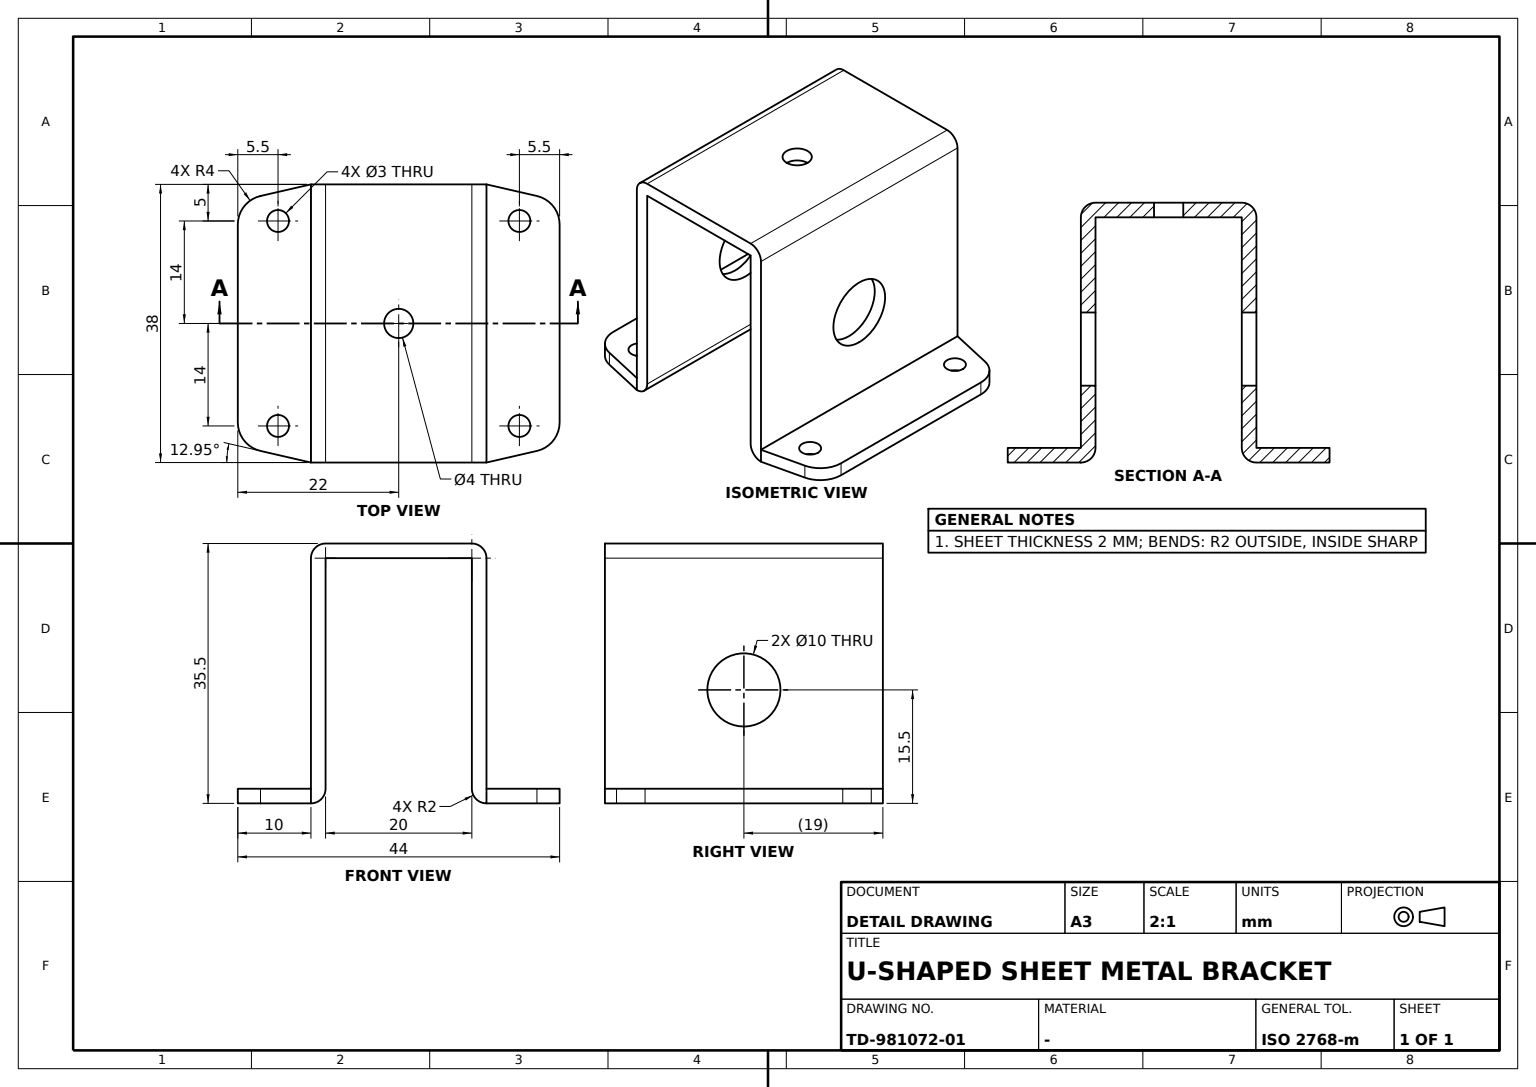
ISO-10303-21;
HEADER;
FILE_DESCRIPTION((''),'2;1');
FILE_NAME('','',(''),(''),'','','');
FILE_SCHEMA(('AUTOMOTIVE_DESIGN'));
ENDSEC;
DATA;
#1=APPLICATION_CONTEXT('');
#2=PRODUCT_CONTEXT('',#1,'mechanical');
#3=PRODUCT('','','',(#2));
#4=PRODUCT_DEFINITION_FORMATION('','',#3);
#5=PRODUCT_DEFINITION_CONTEXT('',#1,'design');
#6=PRODUCT_DEFINITION('','',#4,#5);
#7=PRODUCT_DEFINITION_SHAPE('','',#6);
#8=(LENGTH_UNIT()NAMED_UNIT(*)SI_UNIT(.MILLI.,.METRE.));
#9=(NAMED_UNIT(*)PLANE_ANGLE_UNIT()SI_UNIT($,.RADIAN.));
#10=(NAMED_UNIT(*)SI_UNIT($,.STERADIAN.)SOLID_ANGLE_UNIT());
#11=UNCERTAINTY_MEASURE_WITH_UNIT(LENGTH_MEASURE(0.005),#8,'distance_accuracy_value','');
#12=(GEOMETRIC_REPRESENTATION_CONTEXT(3)GLOBAL_UNCERTAINTY_ASSIGNED_CONTEXT((#11))GLOBAL_UNIT_ASSIGNED_CONTEXT((#8,#9,#10))REPRESENTATION_CONTEXT('',''));
#13=CARTESIAN_POINT('',(-19.,-10.,-31.5));
#14=VERTEX_POINT('',#13);
#15=CARTESIAN_POINT('',(19.,-10.,-31.5));
#16=VERTEX_POINT('',#15);
#17=CARTESIAN_POINT('',(0.,-10.,-31.5));
#18=DIRECTION('',(-1.,0.,0.));
#19=VECTOR('',#18,1000.);
#20=LINE('',#17,#19);
#21=EDGE_CURVE('',#14,#16,#20,.F.);
#22=ORIENTED_EDGE('',*,*,#21,.F.);
#23=CARTESIAN_POINT('',(-19.,-10.,0.));
#24=VERTEX_POINT('',#23);
#25=CARTESIAN_POINT('',(-19.,-10.,2.));
#26=DIRECTION('',(0.,0.,1.));
#27=VECTOR('',#26,1000.);
#28=LINE('',#25,#27);
#29=EDGE_CURVE('',#24,#14,#28,.F.);
#30=ORIENTED_EDGE('',*,*,#29,.F.);
#31=CARTESIAN_POINT('',(19.,-10.,0.));
#32=VERTEX_POINT('',#31);
#33=CARTESIAN_POINT('',(0.,-10.,0.));
#34=DIRECTION('',(1.,0.,0.));
#35=VECTOR('',#34,1000.);
#36=LINE('',#33,#35);
#37=EDGE_CURVE('',#24,#32,#36,.T.);
#38=ORIENTED_EDGE('',*,*,#37,.T.);
#39=CARTESIAN_POINT('',(19.,-10.,2.));
#40=DIRECTION('',(0.,0.,-1.));
#41=VECTOR('',#40,1000.);
#42=LINE('',#39,#41);
#43=EDGE_CURVE('',#32,#16,#42,.T.);
#44=ORIENTED_EDGE('',*,*,#43,.T.);
#45=EDGE_LOOP('',(#22,#30,#38,#44));
#46=FACE_BOUND('',#45,.T.);
#47=CARTESIAN_POINT('',(0.,-10.,-23.));
#48=VERTEX_POINT('',#47);
#49=CARTESIAN_POINT('',(0.,-10.,-18.));
#50=DIRECTION('',(0.,-1.,0.));
#51=AXIS2_PLACEMENT_3D('',#49,#50,#40);
#52=CIRCLE('',#51,5.);
#53=EDGE_CURVE('',#48,#48,#52,.T.);
#54=ORIENTED_EDGE('',*,*,#53,.T.);
#55=EDGE_LOOP('',(#54));
#56=FACE_BOUND('',#55,.T.);
#57=CARTESIAN_POINT('',(0.,-10.,2.));
#58=AXIS2_PLACEMENT_3D('',#57,#50,#18);
#59=PLANE('',#58);
#60=ADVANCED_FACE('',(#46,#56),#59,.F.);
#61=CARTESIAN_POINT('',(-19.,-12.,0.));
#62=VERTEX_POINT('',#61);
#63=VERTEX_POINT('',#25);
#64=AXIS2_PLACEMENT_3D('',#23,#34,#40);
#65=CIRCLE('',#64,2.);
#66=EDGE_CURVE('',#62,#63,#65,.F.);
#67=ORIENTED_EDGE('',*,*,#66,.F.);
#68=CARTESIAN_POINT('',(19.,-12.,0.));
#69=VERTEX_POINT('',#68);
#70=CARTESIAN_POINT('',(0.,-12.,0.));
#71=LINE('',#70,#35);
#72=EDGE_CURVE('',#69,#62,#71,.F.);
#73=ORIENTED_EDGE('',*,*,#72,.F.);
#74=VERTEX_POINT('',#39);
#75=AXIS2_PLACEMENT_3D('',#31,#18,#26);
#76=CIRCLE('',#75,2.);
#77=EDGE_CURVE('',#69,#74,#76,.T.);
#78=ORIENTED_EDGE('',*,*,#77,.T.);
#79=LINE('',#57,#35);
#80=EDGE_CURVE('',#74,#63,#79,.F.);
#81=ORIENTED_EDGE('',*,*,#80,.T.);
#82=EDGE_LOOP('',(#67,#73,#78,#81));
#83=FACE_BOUND('',#82,.T.);
#84=AXIS2_PLACEMENT_3D('',#33,#34,#50);
#85=CYLINDRICAL_SURFACE('',#84,2.);
#86=ADVANCED_FACE('',(#83),#85,.T.);
#87=CARTESIAN_POINT('',(0.,-12.,-23.));
#88=VERTEX_POINT('',#87);
#89=CARTESIAN_POINT('',(0.,-12.,-18.));
#90=AXIS2_PLACEMENT_3D('',#89,#50,#40);
#91=CIRCLE('',#90,5.);
#92=EDGE_CURVE('',#88,#88,#91,.T.);
#93=ORIENTED_EDGE('',*,*,#92,.T.);
#94=EDGE_LOOP('',(#93));
#95=FACE_BOUND('',#94,.T.);
#96=ORIENTED_EDGE('',*,*,#53,.F.);
#97=EDGE_LOOP('',(#96));
#98=FACE_BOUND('',#97,.T.);
#99=CARTESIAN_POINT('',(0.,11.,-18.));
#100=AXIS2_PLACEMENT_3D('',#99,#50,#34);
#101=CYLINDRICAL_SURFACE('',#100,5.);
#102=ADVANCED_FACE('',(#95,#98),#101,.F.);
#103=CARTESIAN_POINT('',(-14.,-15.,-31.5));
#104=VERTEX_POINT('',#103);
#105=CARTESIAN_POINT('',(-14.,-16.5,-31.5));
#106=DIRECTION('',(0.,1.,0.));
#107=AXIS2_PLACEMENT_3D('',#105,#40,#106);
#108=CIRCLE('',#107,1.5);
#109=EDGE_CURVE('',#104,#104,#108,.T.);
#110=ORIENTED_EDGE('',*,*,#109,.F.);
#111=EDGE_LOOP('',(#110));
#112=FACE_BOUND('',#111,.T.);
#113=CARTESIAN_POINT('',(-14.,-15.,-33.5));
#114=VERTEX_POINT('',#113);
#115=CARTESIAN_POINT('',(-14.,-16.5,-33.5));
#116=AXIS2_PLACEMENT_3D('',#115,#40,#106);
#117=CIRCLE('',#116,1.5);
#118=EDGE_CURVE('',#114,#114,#117,.T.);
#119=ORIENTED_EDGE('',*,*,#118,.T.);
#120=EDGE_LOOP('',(#119));
#121=FACE_BOUND('',#120,.T.);
#122=CYLINDRICAL_SURFACE('',#107,1.5);
#123=ADVANCED_FACE('',(#112,#121),#122,.F.);
#124=CARTESIAN_POINT('',(-19.,-12.,-33.5));
#125=VERTEX_POINT('',#124);
#126=CARTESIAN_POINT('',(-19.,-12.,-31.5));
#127=VERTEX_POINT('',#126);
#128=LINE('',#126,#27);
#129=EDGE_CURVE('',#125,#127,#128,.T.);
#130=ORIENTED_EDGE('',*,*,#129,.F.);
#131=CARTESIAN_POINT('',(-17.413784,-18.896591,-33.5));
#132=VERTEX_POINT('',#131);
#133=CARTESIAN_POINT('',(-24.242663,10.794187,-33.5));
#134=DIRECTION('',(-0.224147693,0.974555187,0.));
#135=VECTOR('',#134,1000.);
#136=LINE('',#133,#135);
#137=EDGE_CURVE('',#132,#125,#136,.T.);
#138=ORIENTED_EDGE('',*,*,#137,.F.);
#139=CARTESIAN_POINT('',(-17.413784,-18.896591,-31.5));
#140=VERTEX_POINT('',#139);
#141=LINE('',#131,#41);
#142=EDGE_CURVE('',#132,#140,#141,.F.);
#143=ORIENTED_EDGE('',*,*,#142,.T.);
#144=CARTESIAN_POINT('',(-24.242663,10.794187,-31.5));
#145=LINE('',#144,#135);
#146=EDGE_CURVE('',#140,#127,#145,.T.);
#147=ORIENTED_EDGE('',*,*,#146,.T.);
#148=EDGE_LOOP('',(#130,#138,#143,#147));
#149=FACE_BOUND('',#148,.T.);
#150=CARTESIAN_POINT('',(-17.85,-17.,-31.5));
#151=DIRECTION('',(-0.974555187,-0.224147693,0.));
#152=DIRECTION('',(0.224147693,-0.974555187,0.));
#153=AXIS2_PLACEMENT_3D('',#150,#151,#152);
#154=PLANE('',#153);
#155=ADVANCED_FACE('',(#149),#154,.T.);
#156=CARTESIAN_POINT('',(14.,-15.,-31.5));
#157=VERTEX_POINT('',#156);
#158=CARTESIAN_POINT('',(14.,-16.5,-31.5));
#159=AXIS2_PLACEMENT_3D('',#158,#40,#106);
#160=CIRCLE('',#159,1.5);
#161=EDGE_CURVE('',#157,#157,#160,.F.);
#162=ORIENTED_EDGE('',*,*,#161,.T.);
#163=EDGE_LOOP('',(#162));
#164=FACE_BOUND('',#163,.T.);
#165=CARTESIAN_POINT('',(14.,-15.,-33.5));
#166=VERTEX_POINT('',#165);
#167=CARTESIAN_POINT('',(14.,-16.5,-33.5));
#168=AXIS2_PLACEMENT_3D('',#167,#40,#106);
#169=CIRCLE('',#168,1.5);
#170=EDGE_CURVE('',#166,#166,#169,.F.);
#171=ORIENTED_EDGE('',*,*,#170,.F.);
#172=EDGE_LOOP('',(#171));
#173=FACE_BOUND('',#172,.T.);
#174=CYLINDRICAL_SURFACE('',#159,1.5);
#175=ADVANCED_FACE('',(#164,#173),#174,.F.);
#176=CARTESIAN_POINT('',(13.515563,22.,-33.5));
#177=VERTEX_POINT('',#176);
#178=CARTESIAN_POINT('',(-13.515563,22.,-33.5));
#179=VERTEX_POINT('',#178);
#180=CARTESIAN_POINT('',(-19.,22.,-33.5));
#181=LINE('',#180,#19);
#182=EDGE_CURVE('',#177,#179,#181,.T.);
#183=ORIENTED_EDGE('',*,*,#182,.F.);
#184=CARTESIAN_POINT('',(17.413784,18.896591,-33.5));
#185=VERTEX_POINT('',#184);
#186=CARTESIAN_POINT('',(13.515563,18.,-33.5));
#187=AXIS2_PLACEMENT_3D('',#186,#40,#106);
#188=CIRCLE('',#187,4.);
#189=EDGE_CURVE('',#185,#177,#188,.F.);
#190=ORIENTED_EDGE('',*,*,#189,.F.);
#191=CARTESIAN_POINT('',(19.,12.,-33.5));
#192=VERTEX_POINT('',#191);
#193=CARTESIAN_POINT('',(17.090797,20.300883,-33.5));
#194=VECTOR('',#152,1000.);
#195=LINE('',#193,#194);
#196=EDGE_CURVE('',#185,#192,#195,.T.);
#197=ORIENTED_EDGE('',*,*,#196,.T.);
#198=CARTESIAN_POINT('',(-19.,12.,-33.5));
#199=VERTEX_POINT('',#198);
#200=CARTESIAN_POINT('',(0.,12.,-33.5));
#201=LINE('',#200,#35);
#202=EDGE_CURVE('',#199,#192,#201,.T.);
#203=ORIENTED_EDGE('',*,*,#202,.F.);
#204=CARTESIAN_POINT('',(-17.413784,18.896591,-33.5));
#205=VERTEX_POINT('',#204);
#206=DIRECTION('',(-0.224147693,-0.974555187,0.));
#207=VECTOR('',#206,1000.);
#208=LINE('',#198,#207);
#209=EDGE_CURVE('',#205,#199,#208,.T.);
#210=ORIENTED_EDGE('',*,*,#209,.F.);
#211=CARTESIAN_POINT('',(-13.515563,18.,-33.5));
#212=AXIS2_PLACEMENT_3D('',#211,#40,#106);
#213=CIRCLE('',#212,4.);
#214=EDGE_CURVE('',#179,#205,#213,.F.);
#215=ORIENTED_EDGE('',*,*,#214,.F.);
#216=EDGE_LOOP('',(#183,#190,#197,#203,#210,#215));
#217=FACE_BOUND('',#216,.T.);
#218=CARTESIAN_POINT('',(-14.,18.,-33.5));
#219=VERTEX_POINT('',#218);
#220=CARTESIAN_POINT('',(-14.,16.5,-33.5));
#221=AXIS2_PLACEMENT_3D('',#220,#40,#106);
#222=CIRCLE('',#221,1.5);
#223=EDGE_CURVE('',#219,#219,#222,.F.);
#224=ORIENTED_EDGE('',*,*,#223,.T.);
#225=EDGE_LOOP('',(#224));
#226=FACE_BOUND('',#225,.T.);
#227=CARTESIAN_POINT('',(14.,18.,-33.5));
#228=VERTEX_POINT('',#227);
#229=CARTESIAN_POINT('',(14.,16.5,-33.5));
#230=AXIS2_PLACEMENT_3D('',#229,#40,#106);
#231=CIRCLE('',#230,1.5);
#232=EDGE_CURVE('',#228,#228,#231,.T.);
#233=ORIENTED_EDGE('',*,*,#232,.F.);
#234=EDGE_LOOP('',(#233));
#235=FACE_BOUND('',#234,.T.);
#236=AXIS2_PLACEMENT_3D('',#198,#40,#106);
#237=PLANE('',#236);
#238=ADVANCED_FACE('',(#217,#226,#235),#237,.T.);
#239=CARTESIAN_POINT('',(0.,10.,-23.));
#240=VERTEX_POINT('',#239);
#241=CARTESIAN_POINT('',(0.,10.,-18.));
#242=AXIS2_PLACEMENT_3D('',#241,#50,#40);
#243=CIRCLE('',#242,5.);
#244=EDGE_CURVE('',#240,#240,#243,.T.);
#245=ORIENTED_EDGE('',*,*,#244,.T.);
#246=EDGE_LOOP('',(#245));
#247=FACE_BOUND('',#246,.T.);
#248=CARTESIAN_POINT('',(0.,12.,-23.));
#249=VERTEX_POINT('',#248);
#250=CARTESIAN_POINT('',(0.,12.,-18.));
#251=AXIS2_PLACEMENT_3D('',#250,#50,#40);
#252=CIRCLE('',#251,5.);
#253=EDGE_CURVE('',#249,#249,#252,.T.);
#254=ORIENTED_EDGE('',*,*,#253,.F.);
#255=EDGE_LOOP('',(#254));
#256=FACE_BOUND('',#255,.T.);
#257=ADVANCED_FACE('',(#247,#256),#101,.F.);
#258=CARTESIAN_POINT('',(-14.,18.,-31.5));
#259=VERTEX_POINT('',#258);
#260=CARTESIAN_POINT('',(-14.,16.5,-31.5));
#261=AXIS2_PLACEMENT_3D('',#260,#40,#106);
#262=CIRCLE('',#261,1.5);
#263=EDGE_CURVE('',#259,#259,#262,.T.);
#264=ORIENTED_EDGE('',*,*,#263,.F.);
#265=EDGE_LOOP('',(#264));
#266=FACE_BOUND('',#265,.T.);
#267=ORIENTED_EDGE('',*,*,#223,.F.);
#268=EDGE_LOOP('',(#267));
#269=FACE_BOUND('',#268,.T.);
#270=CYLINDRICAL_SURFACE('',#261,1.5);
#271=ADVANCED_FACE('',(#266,#269),#270,.F.);
#272=CARTESIAN_POINT('',(19.,12.,-31.5));
#273=VERTEX_POINT('',#272);
#274=CARTESIAN_POINT('',(19.,12.,-15.75));
#275=LINE('',#274,#41);
#276=EDGE_CURVE('',#192,#273,#275,.F.);
#277=ORIENTED_EDGE('',*,*,#276,.T.);
#278=CARTESIAN_POINT('',(19.,12.,0.));
#279=VERTEX_POINT('',#278);
#280=LINE('',#274,#27);
#281=EDGE_CURVE('',#273,#279,#280,.T.);
#282=ORIENTED_EDGE('',*,*,#281,.T.);
#283=CARTESIAN_POINT('',(19.,10.,2.));
#284=VERTEX_POINT('',#283);
#285=CARTESIAN_POINT('',(19.,10.,0.));
#286=AXIS2_PLACEMENT_3D('',#285,#18,#26);
#287=CIRCLE('',#286,2.);
#288=EDGE_CURVE('',#279,#284,#287,.F.);
#289=ORIENTED_EDGE('',*,*,#288,.T.);
#290=CARTESIAN_POINT('',(19.,12.,2.));
#291=VECTOR('',#106,1000.);
#292=LINE('',#290,#291);
#293=EDGE_CURVE('',#284,#74,#292,.F.);
#294=ORIENTED_EDGE('',*,*,#293,.T.);
#295=ORIENTED_EDGE('',*,*,#77,.F.);
#296=CARTESIAN_POINT('',(19.,-12.,-31.5));
#297=VERTEX_POINT('',#296);
#298=CARTESIAN_POINT('',(19.,-12.,-15.75));
#299=LINE('',#298,#27);
#300=EDGE_CURVE('',#297,#69,#299,.T.);
#301=ORIENTED_EDGE('',*,*,#300,.F.);
#302=CARTESIAN_POINT('',(19.,-12.,-33.5));
#303=VERTEX_POINT('',#302);
#304=LINE('',#298,#41);
#305=EDGE_CURVE('',#303,#297,#304,.F.);
#306=ORIENTED_EDGE('',*,*,#305,.F.);
#307=AXIS2_PLACEMENT_3D('',#296,#18,#26);
#308=CIRCLE('',#307,2.);
#309=EDGE_CURVE('',#16,#303,#308,.T.);
#310=ORIENTED_EDGE('',*,*,#309,.F.);
#311=ORIENTED_EDGE('',*,*,#43,.F.);
#312=VERTEX_POINT('',#285);
#313=LINE('',#278,#291);
#314=EDGE_CURVE('',#312,#32,#313,.F.);
#315=ORIENTED_EDGE('',*,*,#314,.F.);
#316=CARTESIAN_POINT('',(19.,10.,-31.5));
#317=VERTEX_POINT('',#316);
#318=CARTESIAN_POINT('',(19.,10.,-15.75));
#319=LINE('',#318,#27);
#320=EDGE_CURVE('',#317,#312,#319,.T.);
#321=ORIENTED_EDGE('',*,*,#320,.F.);
#322=AXIS2_PLACEMENT_3D('',#272,#18,#26);
#323=CIRCLE('',#322,2.);
#324=EDGE_CURVE('',#317,#192,#323,.F.);
#325=ORIENTED_EDGE('',*,*,#324,.T.);
#326=EDGE_LOOP('',(#277,#282,#289,#294,#295,#301,#306,#310,#311,#315,#321,#325));
#327=FACE_BOUND('',#326,.T.);
#328=AXIS2_PLACEMENT_3D('',#274,#18,#106);
#329=PLANE('',#328);
#330=ADVANCED_FACE('',(#327),#329,.F.);
#331=CARTESIAN_POINT('',(-13.515563,22.,-31.5));
#332=VERTEX_POINT('',#331);
#333=LINE('',#178,#41);
#334=EDGE_CURVE('',#179,#332,#333,.F.);
#335=ORIENTED_EDGE('',*,*,#334,.T.);
#336=CARTESIAN_POINT('',(13.515563,22.,-31.5));
#337=VERTEX_POINT('',#336);
#338=CARTESIAN_POINT('',(0.,22.,-31.5));
#339=LINE('',#338,#35);
#340=EDGE_CURVE('',#332,#337,#339,.T.);
#341=ORIENTED_EDGE('',*,*,#340,.T.);
#342=LINE('',#176,#41);
#343=EDGE_CURVE('',#177,#337,#342,.F.);
#344=ORIENTED_EDGE('',*,*,#343,.F.);
#345=ORIENTED_EDGE('',*,*,#182,.T.);
#346=EDGE_LOOP('',(#335,#341,#344,#345));
#347=FACE_BOUND('',#346,.T.);
#348=CARTESIAN_POINT('',(0.,22.,-33.5));
#349=AXIS2_PLACEMENT_3D('',#348,#50,#34);
#350=PLANE('',#349);
#351=ADVANCED_FACE('',(#347),#350,.F.);
#352=CARTESIAN_POINT('',(-19.,10.,-31.5));
#353=VERTEX_POINT('',#352);
#354=CARTESIAN_POINT('',(0.,10.,-31.5));
#355=LINE('',#354,#35);
#356=EDGE_CURVE('',#353,#317,#355,.T.);
#357=ORIENTED_EDGE('',*,*,#356,.F.);
#358=CARTESIAN_POINT('',(-19.,12.,-31.5));
#359=AXIS2_PLACEMENT_3D('',#358,#34,#40);
#360=CIRCLE('',#359,2.);
#361=EDGE_CURVE('',#353,#199,#360,.T.);
#362=ORIENTED_EDGE('',*,*,#361,.T.);
#363=ORIENTED_EDGE('',*,*,#202,.T.);
#364=ORIENTED_EDGE('',*,*,#324,.F.);
#365=EDGE_LOOP('',(#357,#362,#363,#364));
#366=FACE_BOUND('',#365,.T.);
#367=CARTESIAN_POINT('',(0.,12.,-31.5));
#368=AXIS2_PLACEMENT_3D('',#367,#34,#40);
#369=CYLINDRICAL_SURFACE('',#368,2.);
#370=ADVANCED_FACE('',(#366),#369,.T.);
#371=CARTESIAN_POINT('',(-19.,10.,0.));
#372=VERTEX_POINT('',#371);
#373=CARTESIAN_POINT('',(0.,10.,0.));
#374=LINE('',#373,#35);
#375=EDGE_CURVE('',#372,#312,#374,.T.);
#376=ORIENTED_EDGE('',*,*,#375,.F.);
#377=LINE('',#352,#41);
#378=EDGE_CURVE('',#353,#372,#377,.F.);
#379=ORIENTED_EDGE('',*,*,#378,.F.);
#380=ORIENTED_EDGE('',*,*,#356,.T.);
#381=ORIENTED_EDGE('',*,*,#320,.T.);
#382=EDGE_LOOP('',(#376,#379,#380,#381));
#383=FACE_BOUND('',#382,.T.);
#384=ORIENTED_EDGE('',*,*,#244,.F.);
#385=EDGE_LOOP('',(#384));
#386=FACE_BOUND('',#385,.T.);
#387=CARTESIAN_POINT('',(0.,10.,2.));
#388=AXIS2_PLACEMENT_3D('',#387,#50,#18);
#389=PLANE('',#388);
#390=ADVANCED_FACE('',(#383,#386),#389,.T.);
#391=ORIENTED_EDGE('',*,*,#209,.T.);
#392=VERTEX_POINT('',#358);
#393=LINE('',#358,#27);
#394=EDGE_CURVE('',#199,#392,#393,.T.);
#395=ORIENTED_EDGE('',*,*,#394,.T.);
#396=CARTESIAN_POINT('',(-17.413784,18.896591,-31.5));
#397=VERTEX_POINT('',#396);
#398=LINE('',#358,#207);
#399=EDGE_CURVE('',#397,#392,#398,.T.);
#400=ORIENTED_EDGE('',*,*,#399,.F.);
#401=LINE('',#204,#41);
#402=EDGE_CURVE('',#205,#397,#401,.F.);
#403=ORIENTED_EDGE('',*,*,#402,.F.);
#404=EDGE_LOOP('',(#391,#395,#400,#403));
#405=FACE_BOUND('',#404,.T.);
#406=CARTESIAN_POINT('',(-17.85,17.,-31.5));
#407=DIRECTION('',(0.974555187,-0.224147693,0.));
#408=DIRECTION('',(0.224147693,0.974555187,0.));
#409=AXIS2_PLACEMENT_3D('',#406,#407,#408);
#410=PLANE('',#409);
#411=ADVANCED_FACE('',(#405),#410,.F.);
#412=CARTESIAN_POINT('',(0.,-12.,-31.5));
#413=LINE('',#412,#35);
#414=EDGE_CURVE('',#127,#297,#413,.T.);
#415=ORIENTED_EDGE('',*,*,#414,.T.);
#416=ORIENTED_EDGE('',*,*,#300,.T.);
#417=ORIENTED_EDGE('',*,*,#72,.T.);
#418=LINE('',#126,#41);
#419=EDGE_CURVE('',#127,#62,#418,.F.);
#420=ORIENTED_EDGE('',*,*,#419,.F.);
#421=EDGE_LOOP('',(#415,#416,#417,#420));
#422=FACE_BOUND('',#421,.T.);
#423=ORIENTED_EDGE('',*,*,#92,.F.);
#424=EDGE_LOOP('',(#423));
#425=FACE_BOUND('',#424,.T.);
#426=CARTESIAN_POINT('',(0.,-12.,2.));
#427=AXIS2_PLACEMENT_3D('',#426,#50,#18);
#428=PLANE('',#427);
#429=ADVANCED_FACE('',(#422,#425),#428,.T.);
#430=CARTESIAN_POINT('',(2.,0.,2.));
#431=VERTEX_POINT('',#430);
#432=CARTESIAN_POINT('',(0.,0.,2.));
#433=AXIS2_PLACEMENT_3D('',#432,#26,#34);
#434=CIRCLE('',#433,2.);
#435=EDGE_CURVE('',#431,#431,#434,.T.);
#436=ORIENTED_EDGE('',*,*,#435,.T.);
#437=EDGE_LOOP('',(#436));
#438=FACE_BOUND('',#437,.T.);
#439=CARTESIAN_POINT('',(2.,0.,0.));
#440=VERTEX_POINT('',#439);
#441=CARTESIAN_POINT('',(0.,0.,0.));
#442=AXIS2_PLACEMENT_3D('',#441,#26,#34);
#443=CIRCLE('',#442,2.);
#444=EDGE_CURVE('',#440,#440,#443,.T.);
#445=ORIENTED_EDGE('',*,*,#444,.F.);
#446=EDGE_LOOP('',(#445));
#447=FACE_BOUND('',#446,.T.);
#448=AXIS2_PLACEMENT_3D('',#432,#26,#106);
#449=CYLINDRICAL_SURFACE('',#448,2.);
#450=ADVANCED_FACE('',(#438,#447),#449,.F.);
#451=ORIENTED_EDGE('',*,*,#314,.T.);
#452=ORIENTED_EDGE('',*,*,#37,.F.);
#453=CARTESIAN_POINT('',(-19.,0.,0.));
#454=LINE('',#453,#291);
#455=EDGE_CURVE('',#372,#24,#454,.F.);
#456=ORIENTED_EDGE('',*,*,#455,.F.);
#457=ORIENTED_EDGE('',*,*,#375,.T.);
#458=EDGE_LOOP('',(#451,#452,#456,#457));
#459=FACE_BOUND('',#458,.T.);
#460=ORIENTED_EDGE('',*,*,#444,.T.);
#461=EDGE_LOOP('',(#460));
#462=FACE_BOUND('',#461,.T.);
#463=AXIS2_PLACEMENT_3D('',#441,#26,#106);
#464=PLANE('',#463);
#465=ADVANCED_FACE('',(#459,#462),#464,.F.);
#466=CARTESIAN_POINT('',(13.515563,-22.,-31.5));
#467=VERTEX_POINT('',#466);
#468=CARTESIAN_POINT('',(17.413784,-18.896591,-31.5));
#469=VERTEX_POINT('',#468);
#470=CARTESIAN_POINT('',(13.515563,-18.,-31.5));
#471=AXIS2_PLACEMENT_3D('',#470,#40,#106);
#472=CIRCLE('',#471,4.);
#473=EDGE_CURVE('',#467,#469,#472,.F.);
#474=ORIENTED_EDGE('',*,*,#473,.T.);
#475=CARTESIAN_POINT('',(22.33346,2.493304,-31.5));
#476=VECTOR('',#408,1000.);
#477=LINE('',#475,#476);
#478=EDGE_CURVE('',#469,#297,#477,.T.);
#479=ORIENTED_EDGE('',*,*,#478,.T.);
#480=ORIENTED_EDGE('',*,*,#414,.F.);
#481=ORIENTED_EDGE('',*,*,#146,.F.);
#482=CARTESIAN_POINT('',(-13.515563,-22.,-31.5));
#483=VERTEX_POINT('',#482);
#484=CARTESIAN_POINT('',(-13.515563,-18.,-31.5));
#485=AXIS2_PLACEMENT_3D('',#484,#40,#106);
#486=CIRCLE('',#485,4.);
#487=EDGE_CURVE('',#140,#483,#486,.F.);
#488=ORIENTED_EDGE('',*,*,#487,.T.);
#489=CARTESIAN_POINT('',(-19.,-22.,-31.5));
#490=LINE('',#489,#19);
#491=EDGE_CURVE('',#467,#483,#490,.T.);
#492=ORIENTED_EDGE('',*,*,#491,.F.);
#493=EDGE_LOOP('',(#474,#479,#480,#481,#488,#492));
#494=FACE_BOUND('',#493,.T.);
#495=ORIENTED_EDGE('',*,*,#161,.F.);
#496=EDGE_LOOP('',(#495));
#497=FACE_BOUND('',#496,.T.);
#498=ORIENTED_EDGE('',*,*,#109,.T.);
#499=EDGE_LOOP('',(#498));
#500=FACE_BOUND('',#499,.T.);
#501=AXIS2_PLACEMENT_3D('',#358,#40,#106);
#502=PLANE('',#501);
#503=ADVANCED_FACE('',(#494,#497,#500),#502,.F.);
#504=ORIENTED_EDGE('',*,*,#334,.F.);
#505=ORIENTED_EDGE('',*,*,#214,.T.);
#506=ORIENTED_EDGE('',*,*,#402,.T.);
#507=CARTESIAN_POINT('',(-13.515563,18.,-31.5));
#508=AXIS2_PLACEMENT_3D('',#507,#40,#106);
#509=CIRCLE('',#508,4.);
#510=EDGE_CURVE('',#332,#397,#509,.F.);
#511=ORIENTED_EDGE('',*,*,#510,.F.);
#512=EDGE_LOOP('',(#504,#505,#506,#511));
#513=FACE_BOUND('',#512,.T.);
#514=CYLINDRICAL_SURFACE('',#212,4.);
#515=ADVANCED_FACE('',(#513),#514,.T.);
#516=CARTESIAN_POINT('',(13.515563,-22.,-33.5));
#517=VERTEX_POINT('',#516);
#518=LINE('',#516,#41);
#519=EDGE_CURVE('',#517,#467,#518,.F.);
#520=ORIENTED_EDGE('',*,*,#519,.F.);
#521=CARTESIAN_POINT('',(17.413784,-18.896591,-33.5));
#522=VERTEX_POINT('',#521);
#523=CARTESIAN_POINT('',(13.515563,-18.,-33.5));
#524=AXIS2_PLACEMENT_3D('',#523,#40,#106);
#525=CIRCLE('',#524,4.);
#526=EDGE_CURVE('',#517,#522,#525,.F.);
#527=ORIENTED_EDGE('',*,*,#526,.T.);
#528=LINE('',#521,#41);
#529=EDGE_CURVE('',#522,#469,#528,.F.);
#530=ORIENTED_EDGE('',*,*,#529,.T.);
#531=ORIENTED_EDGE('',*,*,#473,.F.);
#532=EDGE_LOOP('',(#520,#527,#530,#531));
#533=FACE_BOUND('',#532,.T.);
#534=CYLINDRICAL_SURFACE('',#524,4.);
#535=ADVANCED_FACE('',(#533),#534,.T.);
#536=ORIENTED_EDGE('',*,*,#529,.F.);
#537=CARTESIAN_POINT('',(22.33346,2.493304,-33.5));
#538=LINE('',#537,#476);
#539=EDGE_CURVE('',#522,#303,#538,.T.);
#540=ORIENTED_EDGE('',*,*,#539,.T.);
#541=ORIENTED_EDGE('',*,*,#305,.T.);
#542=ORIENTED_EDGE('',*,*,#478,.F.);
#543=EDGE_LOOP('',(#536,#540,#541,#542));
#544=FACE_BOUND('',#543,.T.);
#545=CARTESIAN_POINT('',(17.85,-17.,-31.5));
#546=DIRECTION('',(-0.974555187,0.224147693,0.));
#547=AXIS2_PLACEMENT_3D('',#545,#546,#408);
#548=PLANE('',#547);
#549=ADVANCED_FACE('',(#544),#548,.F.);
#550=ORIENTED_EDGE('',*,*,#263,.T.);
#551=EDGE_LOOP('',(#550));
#552=FACE_BOUND('',#551,.T.);
#553=CARTESIAN_POINT('',(14.,18.,-31.5));
#554=VERTEX_POINT('',#553);
#555=CARTESIAN_POINT('',(14.,16.5,-31.5));
#556=AXIS2_PLACEMENT_3D('',#555,#40,#106);
#557=CIRCLE('',#556,1.5);
#558=EDGE_CURVE('',#554,#554,#557,.T.);
#559=ORIENTED_EDGE('',*,*,#558,.T.);
#560=EDGE_LOOP('',(#559));
#561=FACE_BOUND('',#560,.T.);
#562=CARTESIAN_POINT('',(17.413784,18.896591,-31.5));
#563=VERTEX_POINT('',#562);
#564=CARTESIAN_POINT('',(17.090797,20.300883,-31.5));
#565=LINE('',#564,#194);
#566=EDGE_CURVE('',#563,#273,#565,.T.);
#567=ORIENTED_EDGE('',*,*,#566,.F.);
#568=CARTESIAN_POINT('',(13.515563,18.,-31.5));
#569=AXIS2_PLACEMENT_3D('',#568,#40,#106);
#570=CIRCLE('',#569,4.);
#571=EDGE_CURVE('',#563,#337,#570,.F.);
#572=ORIENTED_EDGE('',*,*,#571,.T.);
#573=ORIENTED_EDGE('',*,*,#340,.F.);
#574=ORIENTED_EDGE('',*,*,#510,.T.);
#575=ORIENTED_EDGE('',*,*,#399,.T.);
#576=LINE('',#358,#19);
#577=EDGE_CURVE('',#273,#392,#576,.T.);
#578=ORIENTED_EDGE('',*,*,#577,.F.);
#579=EDGE_LOOP('',(#567,#572,#573,#574,#575,#578));
#580=FACE_BOUND('',#579,.T.);
#581=ADVANCED_FACE('',(#552,#561,#580),#502,.F.);
#582=CARTESIAN_POINT('',(0.,-12.,-33.5));
#583=LINE('',#582,#19);
#584=EDGE_CURVE('',#125,#303,#583,.F.);
#585=ORIENTED_EDGE('',*,*,#584,.F.);
#586=AXIS2_PLACEMENT_3D('',#126,#34,#40);
#587=CIRCLE('',#586,2.);
#588=EDGE_CURVE('',#14,#125,#587,.F.);
#589=ORIENTED_EDGE('',*,*,#588,.F.);
#590=ORIENTED_EDGE('',*,*,#21,.T.);
#591=ORIENTED_EDGE('',*,*,#309,.T.);
#592=EDGE_LOOP('',(#585,#589,#590,#591));
#593=FACE_BOUND('',#592,.T.);
#594=AXIS2_PLACEMENT_3D('',#412,#18,#40);
#595=CYLINDRICAL_SURFACE('',#594,2.);
#596=ADVANCED_FACE('',(#593),#595,.T.);
#597=ORIENTED_EDGE('',*,*,#343,.T.);
#598=ORIENTED_EDGE('',*,*,#571,.F.);
#599=LINE('',#184,#41);
#600=EDGE_CURVE('',#185,#563,#599,.F.);
#601=ORIENTED_EDGE('',*,*,#600,.F.);
#602=ORIENTED_EDGE('',*,*,#189,.T.);
#603=EDGE_LOOP('',(#597,#598,#601,#602));
#604=FACE_BOUND('',#603,.T.);
#605=CYLINDRICAL_SURFACE('',#187,4.);
#606=ADVANCED_FACE('',(#604),#605,.T.);
#607=ORIENTED_EDGE('',*,*,#435,.F.);
#608=EDGE_LOOP('',(#607));
#609=FACE_BOUND('',#608,.T.);
#610=CARTESIAN_POINT('',(-19.,10.,2.));
#611=VERTEX_POINT('',#610);
#612=CARTESIAN_POINT('',(-19.,0.,2.));
#613=LINE('',#612,#291);
#614=EDGE_CURVE('',#611,#63,#613,.F.);
#615=ORIENTED_EDGE('',*,*,#614,.T.);
#616=ORIENTED_EDGE('',*,*,#80,.F.);
#617=ORIENTED_EDGE('',*,*,#293,.F.);
#618=LINE('',#387,#19);
#619=EDGE_CURVE('',#284,#611,#618,.T.);
#620=ORIENTED_EDGE('',*,*,#619,.T.);
#621=EDGE_LOOP('',(#615,#616,#617,#620));
#622=FACE_BOUND('',#621,.T.);
#623=PLANE('',#448);
#624=ADVANCED_FACE('',(#609,#622),#623,.T.);
#625=ORIENTED_EDGE('',*,*,#519,.T.);
#626=ORIENTED_EDGE('',*,*,#491,.T.);
#627=CARTESIAN_POINT('',(-13.515563,-22.,-33.5));
#628=VERTEX_POINT('',#627);
#629=LINE('',#627,#41);
#630=EDGE_CURVE('',#628,#483,#629,.F.);
#631=ORIENTED_EDGE('',*,*,#630,.F.);
#632=CARTESIAN_POINT('',(-19.,-22.,-33.5));
#633=LINE('',#632,#19);
#634=EDGE_CURVE('',#517,#628,#633,.T.);
#635=ORIENTED_EDGE('',*,*,#634,.F.);
#636=EDGE_LOOP('',(#625,#626,#631,#635));
#637=FACE_BOUND('',#636,.T.);
#638=CARTESIAN_POINT('',(0.,-22.,-33.5));
#639=AXIS2_PLACEMENT_3D('',#638,#50,#34);
#640=PLANE('',#639);
#641=ADVANCED_FACE('',(#637),#640,.T.);
#642=ORIENTED_EDGE('',*,*,#630,.T.);
#643=ORIENTED_EDGE('',*,*,#487,.F.);
#644=ORIENTED_EDGE('',*,*,#142,.F.);
#645=CARTESIAN_POINT('',(-13.515563,-18.,-33.5));
#646=AXIS2_PLACEMENT_3D('',#645,#40,#106);
#647=CIRCLE('',#646,4.);
#648=EDGE_CURVE('',#132,#628,#647,.F.);
#649=ORIENTED_EDGE('',*,*,#648,.T.);
#650=EDGE_LOOP('',(#642,#643,#644,#649));
#651=FACE_BOUND('',#650,.T.);
#652=CYLINDRICAL_SURFACE('',#646,4.);
#653=ADVANCED_FACE('',(#651),#652,.T.);
#654=ORIENTED_EDGE('',*,*,#558,.F.);
#655=EDGE_LOOP('',(#654));
#656=FACE_BOUND('',#655,.T.);
#657=ORIENTED_EDGE('',*,*,#232,.T.);
#658=EDGE_LOOP('',(#657));
#659=FACE_BOUND('',#658,.T.);
#660=CYLINDRICAL_SURFACE('',#556,1.5);
#661=ADVANCED_FACE('',(#656,#659),#660,.F.);
#662=ORIENTED_EDGE('',*,*,#118,.F.);
#663=EDGE_LOOP('',(#662));
#664=FACE_BOUND('',#663,.T.);
#665=ORIENTED_EDGE('',*,*,#526,.F.);
#666=ORIENTED_EDGE('',*,*,#634,.T.);
#667=ORIENTED_EDGE('',*,*,#648,.F.);
#668=ORIENTED_EDGE('',*,*,#137,.T.);
#669=ORIENTED_EDGE('',*,*,#584,.T.);
#670=ORIENTED_EDGE('',*,*,#539,.F.);
#671=EDGE_LOOP('',(#665,#666,#667,#668,#669,#670));
#672=FACE_BOUND('',#671,.T.);
#673=ORIENTED_EDGE('',*,*,#170,.T.);
#674=EDGE_LOOP('',(#673));
#675=FACE_BOUND('',#674,.T.);
#676=ADVANCED_FACE('',(#664,#672,#675),#237,.T.);
#677=ORIENTED_EDGE('',*,*,#196,.F.);
#678=ORIENTED_EDGE('',*,*,#600,.T.);
#679=ORIENTED_EDGE('',*,*,#566,.T.);
#680=ORIENTED_EDGE('',*,*,#276,.F.);
#681=EDGE_LOOP('',(#677,#678,#679,#680));
#682=FACE_BOUND('',#681,.T.);
#683=CARTESIAN_POINT('',(17.85,17.,-31.5));
#684=DIRECTION('',(0.974555187,0.224147693,0.));
#685=AXIS2_PLACEMENT_3D('',#683,#684,#152);
#686=PLANE('',#685);
#687=ADVANCED_FACE('',(#682),#686,.T.);
#688=CARTESIAN_POINT('',(-19.,12.,0.));
#689=VERTEX_POINT('',#688);
#690=CARTESIAN_POINT('',(0.,12.,0.));
#691=LINE('',#690,#19);
#692=EDGE_CURVE('',#279,#689,#691,.T.);
#693=ORIENTED_EDGE('',*,*,#692,.T.);
#694=AXIS2_PLACEMENT_3D('',#371,#34,#40);
#695=CIRCLE('',#694,2.);
#696=EDGE_CURVE('',#689,#611,#695,.T.);
#697=ORIENTED_EDGE('',*,*,#696,.T.);
#698=ORIENTED_EDGE('',*,*,#619,.F.);
#699=ORIENTED_EDGE('',*,*,#288,.F.);
#700=EDGE_LOOP('',(#693,#697,#698,#699));
#701=FACE_BOUND('',#700,.T.);
#702=AXIS2_PLACEMENT_3D('',#373,#18,#106);
#703=CYLINDRICAL_SURFACE('',#702,2.);
#704=ADVANCED_FACE('',(#701),#703,.T.);
#705=LINE('',#358,#41);
#706=EDGE_CURVE('',#392,#689,#705,.F.);
#707=ORIENTED_EDGE('',*,*,#706,.F.);
#708=ORIENTED_EDGE('',*,*,#394,.F.);
#709=ORIENTED_EDGE('',*,*,#361,.F.);
#710=ORIENTED_EDGE('',*,*,#378,.T.);
#711=ORIENTED_EDGE('',*,*,#455,.T.);
#712=ORIENTED_EDGE('',*,*,#29,.T.);
#713=ORIENTED_EDGE('',*,*,#588,.T.);
#714=ORIENTED_EDGE('',*,*,#129,.T.);
#715=ORIENTED_EDGE('',*,*,#419,.T.);
#716=ORIENTED_EDGE('',*,*,#66,.T.);
#717=ORIENTED_EDGE('',*,*,#614,.F.);
#718=ORIENTED_EDGE('',*,*,#696,.F.);
#719=EDGE_LOOP('',(#707,#708,#709,#710,#711,#712,#713,#714,#715,#716,#717,#718));
#720=FACE_BOUND('',#719,.T.);
#721=DIRECTION('',(0.,0.382683432,-0.923879533));
#722=AXIS2_PLACEMENT_3D('',#352,#34,#721);
#723=PLANE('',#722);
#724=ADVANCED_FACE('',(#720),#723,.F.);
#725=ORIENTED_EDGE('',*,*,#253,.T.);
#726=EDGE_LOOP('',(#725));
#727=FACE_BOUND('',#726,.T.);
#728=ORIENTED_EDGE('',*,*,#577,.T.);
#729=ORIENTED_EDGE('',*,*,#706,.T.);
#730=ORIENTED_EDGE('',*,*,#692,.F.);
#731=ORIENTED_EDGE('',*,*,#281,.F.);
#732=EDGE_LOOP('',(#728,#729,#730,#731));
#733=FACE_BOUND('',#732,.T.);
#734=CARTESIAN_POINT('',(0.,12.,2.));
#735=AXIS2_PLACEMENT_3D('',#734,#50,#18);
#736=PLANE('',#735);
#737=ADVANCED_FACE('',(#727,#733),#736,.F.);
#738=CLOSED_SHELL('',(#60,#86,#102,#123,#155,#175,#238,#257,#271,#330,#351,#370,#390,#411,#429,#450,#465,#503,#515,#535,#549,#581,#596,#606,#624,#641,#653,#661,#676,#687,#704,#724,#737));
#739=MANIFOLD_SOLID_BREP('',#738);
#740=ADVANCED_BREP_SHAPE_REPRESENTATION('',(#739),#12);
#741=SHAPE_DEFINITION_REPRESENTATION(#7,#740);
ENDSEC;
END-ISO-10303-21;
